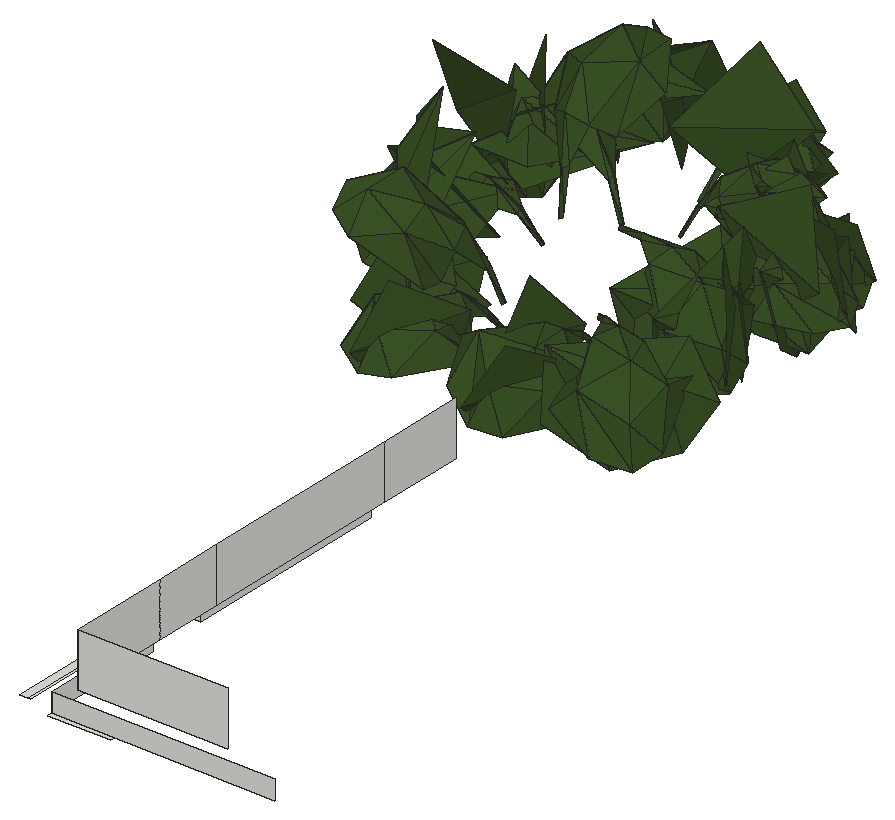
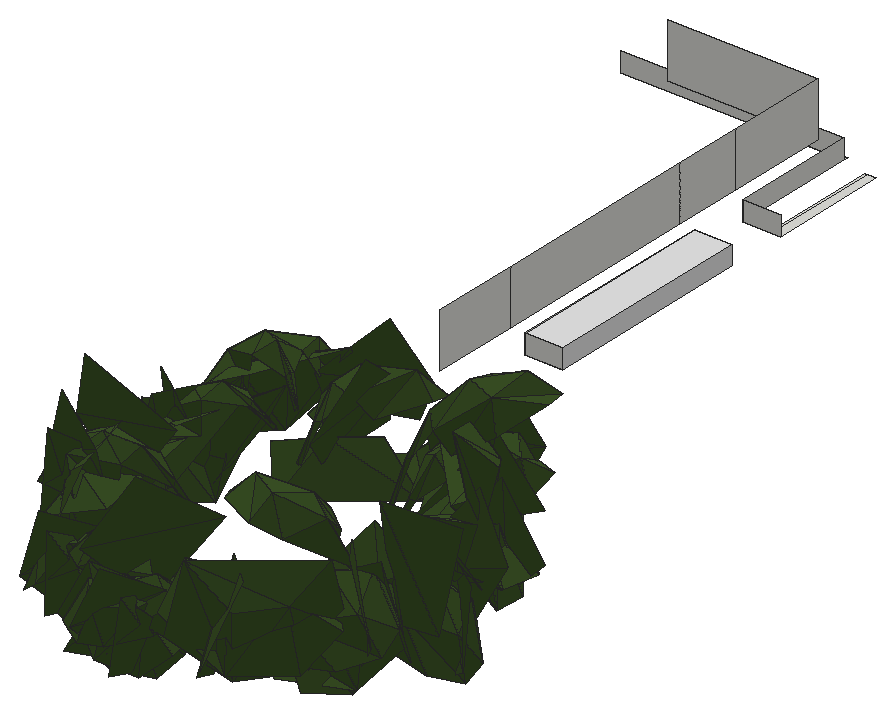
# SketchUp Ruby script. Lengths in inches.
U = 1.inch
M = Sketchup.active_model
def pt(a) = Geom::Point3d.new(a.map { |v| v * U })
def face(e, loops, mat)
  f = e.add_face(loops[0].map { |a| pt(a) })
  loops[1..].each { |l| e.add_face(l.map { |a| pt(a) }).erase! }
  f.material = f.back_material = mat if mat
  f
end
# faces: each face lists its corners as indices into pts; further lists are holes
def faces(e, pts, list, mat = nil) = list.each { |f| face(e, (f[0].is_a?(Array) ? f : [f]).map { |l| l.map { |i| pts[i] } }, mat) }
# xy, xz, yz: faces in a plane at the given z, y or x. An outline is a flat list of corners, or four numbers for a rectangle; further outlines are holes
def ring(l) = l.size == 4 ? [[l[0], l[1]], [l[2], l[1]], [l[2], l[3]], [l[0], l[3]]] : l.each_slice(2).to_a
def flat(e, list, mat, &to3) = list.each { |f| face(e, (f[0].is_a?(Array) ? f : [f]).map { |l| ring(l).map { |u, v| to3.(u, v) } }, mat) }
def xy(e, z, list, mat = nil) = flat(e, list, mat) { |x, y| [x, y, z] }
def xz(e, y, list, mat = nil) = flat(e, list, mat) { |x, z| [x, y, z] }
def yz(e, x, list, mat = nil) = flat(e, list, mat) { |y, z| [x, y, z] }
def lines(e, pts, list) = list.each { |a, b| e.add_line(pt(pts[a]), pt(pts[b])) }
# prism: a flat outline (further loops are holes) pulled along v
def prism(e, loops, v, mat = nil)
  f = face(e, loops, mat); d = Geom::Vector3d.new(v.map { |x| x * U })
  f.pushpull(f.normal.samedirection?(d) ? d.length : -d.length)
end
def box(e, o, s, mat = nil) = prism(e, [[o, [o[0] + s[0], o[1], o[2]], [o[0] + s[0], o[1] + s[1], o[2]], [o[0], o[1] + s[1], o[2]]]], [0, 0, s[2]], mat)
def at(x, y, z, deg = 0) = Geom::Transformation.translation(pt([x, y, z])) * Geom::Transformation.rotation(ORIGIN, Z_AXIS, deg.degrees)
def axes(o, x, y, z) = Geom::Transformation.new([*x, 0, *y, 0, *z, 0, *pt(o).to_a, 1])
def part(name) = M.definitions.add(name)
# library, detail: a bought-in or finely detailed component or shape, given as its bounding box
def library(name, o, s) = part(name).tap { |d| box(d.entities, o, s) }
def detail(e, o, s) = box(e.add_group.entities, o, s)
def put(e, d, t, mat = nil) = e.add_instance(d, t).tap { |i| i.material = mat if mat }
def group(e, t, mat = nil) = e.add_group.tap { |g| g.transformation = t; g.material = mat if mat }.entities
root = M.entities
M.materials.add("AM113_062_Tilia").color = [58, 81, 37]
M.materials.add("white_wall").color = [233, 233, 233]
xy(root,500.91,[[418.81,115.3125,496.21,121.6875],[371.87,130.3125,382.06,278.26],[382.06,130.3125,385.62,278.26]])
xy(root,500.91,[[371.87,353.16,418.81,615.47]],"white_wall")
xy(root,525.1,[[371.87,353.16,418.81,615.47]],"white_wall")
xz(root,121.6875,[[418.81,500.91,695.48,525.1]])
xz(root,139.5,[[436.99,525.1,622.42,592.47]])
xz(root,278.26,[[371.87,500.91,418.81,525.1]])
xz(root,353.16,[[371.87,500.91,418.81,525.1]],"white_wall")
xz(root,615.47,[[371.87,500.91,418.81,525.1]])
yz(root,371.87,[[353.16,500.91,615.47,525.1]],"white_wall")
yz(root,418.81,[[121.6875,500.91,278.26,525.1],[353.16,500.91,615.47,525.1]])
yz(root,436.99,[[139.5,525.1,266.01,592.47],[266.01,525.1,353.16,592.47],[353.16,525.1,615.47,592.47],[615.47,525.1,725.65,592.47]])
p = [[447.91,850.1875,601.09],[480.87,802.46,545.55],[524.63,854.63,485.78],[519.66,855.77,573.08],[550.76,903.55,570.88],[566.41,915.91,493.375],
  [66.82,1152.99,507.09],[97.15,1146.97,487.25],[148.3,1081.53,542.29],[70.04,1143.02,489.34],[77.07,1108.81,493.43],[83.87,1137.56,535.27],
  [126.11,1173.27,559.43],[89.64,1179.86,507.09],[141.26,1229.85,490.56],[139.06,1157.11,521.98],[139.59,1190.19,597.74],[133.73,1250.28,579.96],
  [181.97,1298.85,597.52],[140.7,1312.06,529.03],[460.33,1197.81,509.56],[504.98,1203.63,490.94],[506.78,1216.99,523.57],[521.83,1250.84,491.55],
  [530.97,1079.69,610.26],[563.39,1070.9,539.31],[530.76,1136.5,491.14],[554.3125,1134.13,573.8],[530.96,1187.11,581.77],[511.65,1204.9375,507.36],
  [507.98,1282.76,501.61],[176.48,942.12,491.66],[227.05,891.03,499.89],[227.5625,915.73,575.1875],[183.07,953.21,578.2],[189.36,1017.86,590.34],
  [136.96,999.375,548.22],[518.23,1275.49,509.68],[495.63,1265.62,492.5],[438.95,1246.59,552.56],[484.28,1275.96,572],[469.9375,1297.82,492.68],
  [415.61,1273.29,514.75],[584.43,950.18,540.22],[135.1875,1050.68,522.83],[108.03,1086.63,545.74],[350.77,1219.13,560.8],[406.07,1241.46,494.25],
  [455.94,1265.91,543.95],[342.85,1283.12,576.94],[359.62,1325.95,494.31],[374.52,1387.23,525.68],[438.95,962.3,611.65],[482.72,941.64,542.47],
  [494.35,1014.66,495.65],[498.36,1001.99,581.5],[506.32,1058.04,590.46],[507.33,1085.99,517.2],[551.23,1044.6,596.52],[525.07,1058.79,495.72],
  [471.1,1096.48,548.77],[497.1,956.03,600.03],[500.73,949.14,517.51],[474.45,1025.35,496.53],[520.47,1007.79,557.6],[516.65,1062.95,581.15],
  [481.05,1093.45,526.12],[292.87,984.37,497.8],[282.8,955.1875,535.73],[288.81,958.66,537.47],[292.6,957.64,531.31],[295.68,983.59,497.81],
  [295.23,986.83,501.03],[140.7,999.67,630.68],[79.29,1009.55,558.58],[139.35,992.91,498.89],[206.45,1053.27,524.83],[209.82,1078.24,537.58],
  [116.34,1088.94,499.17],[70.63,1078.21,589.95],[413.37,931.5,550.39],[430.11,992.57,499.42],[298.04,925.78,517.78],[472.57,943.125,530.68],
  [266.72,873.6875,541.33],[504.57,1263.71,533.37],[484.96,1291.55,519.97],[212.29,919.98,623.86],[172.99,892.09,535.71],[245.73,899.09,501.97],
  [272.37,985.95,524.2],[383.31,1336.6875,601.39],[399.96,1363.62,549.01],[345.9,1352.99,502.82],[347.39,1366.73,570.93],[288.5,1350.2,508.87],
  [301.66,1358.17,571.11],[119.21,993.93,502.99],[152.05,954.03,522.83],[143.72,999.76,578.03],[98.32,1060.89,524.86],[474.87,1070.72,588.94],
  [540.9,1059.84,553.85],[550.79,1131.46,502.96],[528.22,1123.58,584.89],[519.88,1180,585.72],[539.25,1204.4,514.64],[314.03,857.13,538.16],
  [392.29,855.66,505.11],[363.78,903.56,555.05],[454.3125,896.72,507.18],[125.51,1243.76,505.61],[113.53,1168.99,535.21],[153.61,1193.39,597.49],
  [164.9,1251.9,582.9],[236.2,1283.875,561.15],[169.13,1315.93,536.15],[154.2,1007.49,573.32],[139.42,952.86,539.93],[198.6,978.07,505.88],
  [192.15,1119.27,565.37],[140.41,1071.16,570.82],[77.11,1126.41,588.08],[145.85,1194.83,533.875],[501.82,1240.17,558.45],[507.76,824.62,581.64],
  [535.83,807.78,523.32],[570.46,833.44,508.39],[561.96,839.4375,557.13],[580.59,866.67,518.5],[256.57,1346.67,545.89],[501.45,968.14,582.11],
  [527.71,973.07,518.9],[546.71,1012.75,509.22],[541.58,1007.95,558.95],[543.09,1045.22,527.51],[453.73,1198.22,538.52],[441.48,1247.4375,579.22],
  [509.8,1257.28,577.0625],[412.52,1219.85,602.63],[451.3,1229.27,560.65],[415.82,1268.25,510.05],[416.25,1269.25,580.45],[375.79,1309.71,512.41],
  [380.42,1298.71,575.9],[560.05,1179.21,617.48],[567.94,1182.12,510.15],[494.67,1206.07,521.91],[244.54,801.95,541.64],[250.54,826.95,510.85],
  [313.74,891.83,547.15],[331.65,1233.42,542.69],[318.3125,1223.97,511.11],[316.29,1221.85,513],[332.34,1230.22,547.48],[319.3125,1221.87,511.06],
  [337.7,1228.47,547.0625],[346.8,1328.27,545.82],[162.0625,942.01,514.1],[207.12,883.25,523.55],[234.53,926.86,571.02],[202.77,974.23,570.48],
  [223.35,1041.3125,535.68],[154.67,1020.29,545.73],[552.27,999.05,521.46],[519.29,1009.6,514.2],[483.48,1061.51,605.58],[520.07,1239.02,560.28],
  [352.77,1366.97,514.57],[350.22,1344.01,577.86],[381.28,1292.62,579.47],[403.64,1343.43,559.0625],[304.94,1348.0625,573.64],[293.51,1371.11,517.46],
  [428.91,1203.51,540.99],[419.97,1193.43,539.82],[394.26,1182.37,519.06],[395.92,1183.33,515.47],[424.54,1193.28,535.56],[416.75,1196.5,537.0625],
  [394.6875,1185.0625,516.7],[514.15,1117.94,571.17],[395.73,1300.69,613.09],[361.13,1303.75,517.53],[342.05,1238.18,553.91],[421.06,1312.46,534.79],
  [260.66,1360.5,549.26],[406.07,782.48,524.875],[438.12,796.97,517.66],[415.8,801.8125,567.01],[461.07,837.3125,559.23],[485.6,869.32,522.91],
  [259.96,1266.02,621.1],[241.22,1320.45,517.69],[205.76,1390.97,556.95],[311.06,1377.46,602.9375],[316.23,1389.375,518.39],[283.73,1336.55,518.62],
  [564.89,894.8,578.39],[557.0625,942.12,564.31],[322.49,1287.52,569.46],[475.82,953,556.29],[463.74,1267.42,560.88],[424.9,1272.67,557.1],
  [400.16,778.98,545.73],[395.59,808.17,521.33],[456.04,877.73,550.25],[312.95,905.48,521.39],[307.41,909.36,558.26],[309.48,853.41,565.96],
  [346.03,875.74,534.77],[497.09,1065.1875,633.88],[558.42,1006.97,610.87],[451.05,1141.24,585.71],[145.52,1124.38,582.13],[194.92,971.05,560.45],
  [167,1082.47,523.27],[447.6,894.07,529.97],[479.07,817.625,555.37],[162.4,1086.83,559.67],[220.67,870.87,568.35],[216.7,823.06,531.56],
  [255.18,801.31,523.625],[258.8,825.63,562.98],[289.56,810.36,526.36],[252.24,868.625,554.3],[473.64,1236.38,560],[251.54,1201.92,566.37],
  [277.41,1185.12,527.79],[274.75,1187.21,523.96],[248.26,1208.15,562.98],[375.5625,838.38,597.59],[368.93,795.86,551.74],[123.55,1050.04,605.55],
  [161.14,1101.41,626.16],[100.55,1115.36,604.29],[249.58,1196.96,561.41],[273.68,1184.41,525.01],[338.44,1370.61,601.54],[382.16,1195.58,567.91],
  [437.22,1212.69,564.49],[428.72,1270.74,526.02],[400.25,1252.02,580.4375],[374.69,1289.55,575.46],[393.09,1318.31,527.3125],[497.92,1123.27,579.81],
  [359.11,1333.59,553.46],[523.44,1055.42,594.57],[495.33,1095.78,594.14],[206.23,1335.11,528.33],[153.76,1285.91,535.91],[159.85,1304.18,613.81],
  [196.51,1349.42,613.59],[255.11,1349.89,651.71],[249.16,1389.07,586.14],[242.89,922.77,528.53],[199.15,883.24,534.93],[261.47,929.36,556.48],
  [450.56,892.25,567.59],[300.94,914.56,530.04],[120.22,1213.01,638.51],[92.4,1201.34,530.6],[157.86,1151.12,533.64],[285.36,922.53,571.29],
  [214.26,1100.33,553.33],[246.18,1097.22,531.47],[248.49,1097.46,535.73],[102.42,990.41,531.83],[89.63,1062.06,551.72],[397.21,845.13,585.28],
  [394.17,856.625,542.72],[403.43,950.64,531.88],[405.93,965.66,559.1875],[213.91,1103.86,559.72],[246.98,1099.96,531.9],[211.2,1109.9375,557.1],
  [234.43,1205.14,572.13],[596.16,1132.8,559.74],[567.47,1133.92,533.77],[494.08,1177.83,586.64],[183.36,1150.55,540.33],[424.4,939.91,560.35],
  [416.32,969.85,534.7],[416.26,972.51,538.73],[426.68,1240.52,534.94],[437.26,1231.07,559.06],[128.38,1132.68,587.59],[128.24,1115.27,571.02],
  [446.99,1211.29,559.41],[413.57,970.11,535.88],[416.48,935.25,567.33],[422.15,939.46,567.76],[126.17,1256.67,582.24],[288.81,960.29,578.55],
  [294.4375,975.64,535.96],[296.8,978.73,537.64],[319.11,1274.8,562.03],[316.83,1253.25,536.34],[317.2,1250.75,539.04],[322.125,1274.15,567.01],
  [319.08,1252.64,536.36],[326.91,1276.91,565.49],[292.73,977.96,536.52],[281.54,964.77,586.78],[288.42,963.97,584.94],[139.58,1034.79,635.55],
  [443.28,1125.39,631.84],[511.12,1118.83,539.75],[583.62,1104.83,593.02],[529.04,974.14,584.79],[227.68,1150.03,584.9],[235.65,1140.25,540.24],
  [236.625,1136.35,541.29],[182.75,1131.32,568.05],[356.8,1399.57,564.1],[352.18,1378.83,540.52],[301.89,1327.64,571.92],[230.89,1147.47,590.85],
  [238.53,1140.1,540.72],[235.82,1152.15,593.35],[287.47,912.66,582.71],[90.74,1266.03,574.06],[113.82,1251.11,541.53],[179.77,1185.75,592.33],
  [323.49,891.22,578.33],[268.48,831.82,617.29],[183.19,966.11,542.08],[207.89,923.98,571.57],[174.2,959.89,622.63],[149.48,1028.09,561.62],
  [351.86,1244.66,581.375],[349.64,1265.59,572.9],[217.02,1251.48,546.0625],[179.82,1302.16,542.68],[167.84,1287.87,585.61],[114.57,1290.32,552.01],
  [538.14,1091.83,593.95],[581.26,1101.17,549.85],[592.42,1144.05,543.03],[572.27,1139.95,586.0625],[575.99,1175.04,550.97],[201.45,1354.02,543.05],
  [141.59,1309.92,546.67],[171.17,1297.21,616.98],[217.62,1330.05,622.25],[288.9,1306.23,624.27],[269.03,1372.8,598.73],[408.56,1275.59,610.93],
  [353.05,1273.15,544.59],[380.85,1295.11,590.125],[352.07,1307.71,559.67],[472.66,874.95,575.92],[436.96,802.72,616.24],[174.09,1147.3,658.14],
  [134.53,1171.67,545.81],[57.86,1201.625,571.01],[333.28,1302.43,587.63],[268.74,1327.92,594.18],[303.4375,1223.82,628.03],[347.77,1284.93,546.03],
  [396.03,1334.41,608.96],[224.79,1237.01,580.21],[118.87,1273.17,586.46],[361.8,1227.53,569.41],[319.1875,1295.16,548.27],[435.85,1035.83,626.5],
  [264.1,1305.77,560.77],[404.63,1137.39,549.54],[439.06,1133.04,581.49],[434.5,1137.9375,584.42],[402.06,1138.94,553.375],[378.35,1221.3,549.625],
  [423.72,1214.65,564.44],[416.28,1232.07,592.19],[348.33,1399.59,549.65],[345.46,1381.12,582.05],[376.11,1345.31,588.3125],[379.16,1382.6,557],
  [320.89,1392.28,552.09],[527.74,1069.46,560.36],[433.96,1142.125,578.59],[404.73,1140.3,549.75],[534.04,1182.18,598.9375],[500.76,1213.55,575.59],
  [345.89,850.79,577.12],[148.98,1061.93,594.18],[125.1,1126.9,598.61],[302.63,1316.11,551.92],[307,1313.94,581.53],[305.08,1358.79,585.4],
  [276.04,1340.03,561.28],[87.53,1251.71,559.16],[172.37,1107.69,578.08],[466.76,873.79,573.375],[443.29,995.01,589.86],[279.05,877.82,581.32],
  [184.83,1345.87,651.89],[393.43,1334.72,562.21],[533.84,875.85,602.17],[487.11,1216.65,619.08],[343.8,1298.14,581.08],[358.67,1302.8,558.56],
  [505.79,1022.07,614.51],[432.97,853.76,590.92],[386.53,903.73,632.8],[94.24,1215.87,572.36],[116.32,1252.78,598],[495.66,1186.0625,618.49],
  [569.76,1145.4375,641.81],[420.94,1307.49,568.625],[455.77,1218.04,581.08],[431.1875,899.54,591.14],[478.8125,1102.54,564.95],[202.29,1131.01,589.49],
  [216.77,1216.07,604.16],[199.78,1192.4,599.62],[140.7,1004.65,643.62],[159.27,1051.72,697.53],[114.41,1068.71,642.01],[324.64,1303.85,592.54],
  [478.41,1174.9,563.15],[479.83,1166.98,599.58],[141.34,1198.11,614.71],[158.85,1152.01,592.21],[191.94,1180.06,564.02],[294.02,1328.84,596.76],
  [337.64,1377.47,625.63],[513.41,928.66,564.21],[516.47,918.42,599.5],[450.62,1256.41,573.1875],[471.07,1117.71,595.7],[380.97,897.67,566.1],
  [404.3,903.83,587.52],[423.875,1278.77,595.51],[444.41,1291.42,569.75],[380.5,1263.18,598.5],[62.73,1157.375,670.14],[458.92,1109.3,624.52],
  [228.05,934.74,635.5],[477.26,887.39,603.98],[181.03,1181.78,627.7],[126.78,1252.57,656.33],[277.25,940.91,632.31],[282.8,915.93,618.99],
  [473.64,1141.86,611.99],[497.93,1096.4375,641.11],[171.125,1229.56,617.54],[463.39,931.38,597.95],[435.66,951.6,580.66],[433.59,951.97,585.21],
  [433.65,949.49,580.79],[461.66,920.97,599.91],[462.2,927.34,603.8],[329.47,1339.8125,598.75],[450.25,1007.56,622.8125],[178.86,1148.54,634.89],
  [152.99,1248.65,642.68],[220.4,1165.85,641.75],[197.19,1178.15,630.81],[257.24,871.625,649.35],[286.76,863.85,599.6],[273.5,906.15,585.35],
  [519.22,1146.13,614.41],[166.51,1223.77,600.87],[258.35,959.54,623.63],[461.6,1064.99,593.02],[472.22,1052.59,624.51],[546.125,1139.34,686.85],
  [246.61,1169.9375,633.07],[498.11,902.39,616.19],[207.33,846.56,638.26],[194.87,1194.61,599.58],[178.77,1222.43,668.86],[153.68,1208.9375,617.14],
  [232.29,963.21,607.04],[180.625,959.68,643.96],[200.59,939.88,672.7],[343.87,1313.49,697.67],[464.05,1028.25,637.56],[189.99,1277.78,666.25],
  [252.05,910.74,662.65],[267.75,1222.36,690.4],[265.46,1189.55,619.0625],[295.28,1228.47,661.8],[382.86,1046.72,619.66],[421.86,1031.07,628.9],
  [420.1,1036.43,634.39],[382.23,1048.31,624.66],[418.9,1041.29,629.71],[383.78,1049.47,619.99],[212.82,1201.15,678.12],[175.93,860.29,650.76],
  [203.66,880.67,674.93],[161,901.58,661.06],[262.18,1277.86,687.64],[219.48,1256.17,699.11],[220.42,1292.6,680.53]]
faces(root,p,[[0,1,2],[2,3,0],[4,3,2],[2,5,4],[6,7,8],[9,10,11],[9,11,12],[12,13,9],
  [14,15,16],[16,17,14],[14,17,18],[18,19,14],[20,21,22],[22,21,23],[24,25,26],[26,27,24],
  [28,27,26],[26,29,28],[22,23,30],[31,32,33],[33,34,31],[35,36,31],[31,34,35],[37,38,39],
  [40,41,42],[5,43,4],[10,44,45],[11,10,45],[46,47,48],[49,50,51],[52,53,54],[54,55,52],
  [56,55,54],[54,57,56],[58,59,60],[61,62,63],[63,64,61],[65,64,63],[63,66,65],[67,68,69],
  [70,71,72],[69,72,67],[73,74,75],[73,75,76],[77,78,79],[80,81,82],[80,83,81],[32,84,33],
  [72,69,70],[30,85,22],[30,86,85],[87,88,89],[87,89,90],[91,92,93],[93,94,91],[93,95,96],
  [96,94,93],[97,98,99],[100,97,99],[101,102,103],[103,104,101],[105,104,103],[103,106,105],[82,107,108],
  [108,109,82],[80,109,108],[108,110,80],[111,112,113],[113,114,111],[115,116,111],[111,114,115],[117,118,119],
  [117,119,120],[8,121,6],[121,122,6],[12,123,13],[110,83,80],[29,124,28],[125,126,127],[127,128,125],
  [127,129,128],[95,130,96],[131,132,133],[133,134,131],[133,135,134],[22,136,20],[39,137,37],[137,138,37],
  [139,140,141],[141,142,139],[141,143,144],[144,142,141],[145,146,147],[148,149,150],[151,152,153],[154,153,155],
  [155,156,154],[143,157,144],[153,154,151],[158,159,160],[160,161,158],[162,163,158],[158,161,162],[164,165,166],
  [106,167,105],[168,169,170],[170,171,168],[172,169,168],[168,173,172],[40,42,174],[175,176,177],[177,178,175],
  [179,180,176],[57,181,56],[182,183,184],[182,185,183],[173,186,172],[187,188,189],[189,188,190],[188,191,190],
  [192,193,194],[82,109,80],[195,196,197],[128,129,198],[129,199,198],[195,197,200],[131,201,132],[176,175,179],
  [85,86,202],[86,203,202],[204,205,206],[207,208,209],[209,210,207],[166,211,164],[211,212,164],[145,147,213],
  [15,214,16],[99,98,215],[45,44,216],[190,191,217],[125,218,126],[216,219,45],[220,221,222],[222,223,220],
  [222,224,223],[159,225,160],[136,22,226],[22,85,226],[227,228,229],[229,230,227],[231,232,187],[187,189,231],
  [99,233,100],[100,233,234],[234,235,100],[236,237,228],[238,49,51],[239,240,241],[241,242,239],[243,242,241],
  [241,244,243],[66,245,65],[223,224,209],[224,210,209],[244,246,243],[134,135,247],[135,248,247],[228,227,236],
  [249,250,251],[251,252,249],[249,252,253],[253,254,249],[255,256,220],[220,257,255],[217,258,190],[160,225,259],
  [160,259,162],[260,261,262],[263,208,70],[70,69,263],[264,265,266],[220,256,221],[267,118,117],[268,267,117],
  [269,270,271],[271,272,269],[273,266,274],[274,275,273],[226,85,202],[260,262,276],[277,278,279],[280,123,12],
  [281,282,283],[284,285,202],[202,203,284],[112,286,113],[287,11,45],[12,11,287],[288,175,178],[178,136,288],
  [68,257,263],[263,69,68],[162,161,160],[266,273,264],[289,290,291],[291,283,289],[250,292,251],[293,294,295],
  [296,297,298],[299,298,300],[300,301,299],[302,303,304],[304,295,302],[179,175,288],[288,285,179],[295,304,293],
  [305,77,79],[226,288,136],[283,291,281],[298,299,296],[306,307,308],[4,43,309],[310,311,312],[12,313,280],
  [314,315,316],[317,312,318],[318,319,317],[33,84,320],[312,317,310],[321,322,323],[150,324,148],[324,325,148],
  [326,327,328],[329,326,328],[151,154,330],[330,331,151],[332,333,334],[334,333,335],[336,337,338],[338,339,336],
  [338,340,339],[341,342,343],[343,344,341],[345,346,341],[341,344,345],[347,46,48],[348,331,349],[349,350,348],
  [206,351,204],[351,352,204],[287,45,219],[353,354,355],[144,157,356],[96,130,357],[358,359,360],[334,361,332],
  [342,362,343],[156,363,330],[330,154,156],[243,364,239],[243,246,364],[58,60,365],[172,186,366],[367,368,369],
  [369,370,367],[371,372,373],[373,363,371],[374,375,376],[376,377,374],[374,378,375],[336,379,337],[380,381,370],
  [339,340,382],[340,383,382],[231,384,232],[117,385,268],[268,385,120],[120,386,268],[387,388,389],[389,390,387],
  [334,335,391],[378,390,389],[375,378,389],[392,219,264],[264,273,392],[370,369,380],[393,218,125],[394,201,131],
  [257,220,395],[395,263,257],[396,192,194],[376,397,377],[125,128,398],[398,128,198],[392,273,275],[275,313,392],
  [61,64,65],[395,209,208],[395,208,263],[28,124,399],[376,400,401],[401,397,376],[131,134,402],[402,134,247],
  [226,285,288],[226,202,285],[403,189,190],[403,190,258],[272,404,269],[391,405,406],[391,406,334],[313,12,287],
  [287,219,392],[279,407,277],[407,408,277],[409,350,349],[105,167,410],[411,258,281],[281,291,411],[99,215,234],
  [412,379,336],[172,366,170],[113,413,115],[115,114,113],[414,415,236],[236,227,414],[328,416,329],[329,416,417],
  [417,418,329],[296,299,419],[419,388,296],[220,223,395],[395,223,209],[414,227,230],[230,361,414],[420,421,382],
  [382,383,420],[422,423,424],[424,415,422],[316,425,314],[425,426,314],[198,199,427],[427,428,198],[373,372,429],
  [336,430,412],[120,385,117],[419,299,301],[301,400,419],[431,384,231],[231,432,431],[231,189,403],[290,432,411],
  [411,291,290],[403,258,411],[239,242,243],[287,392,313],[433,409,349],[434,409,433],[435,330,363],[363,373,435],
  [373,429,434],[434,433,373],[4,309,0],[0,3,4],[91,94,96],[436,353,355],[96,357,91],[56,181,437],
  [328,327,438],[405,423,422],[406,405,422],[435,331,330],[435,349,331],[125,439,393],[170,169,172],[24,27,28],
  [323,440,321],[440,441,321],[33,320,35],[35,34,33],[144,356,139],[139,142,144],[234,233,99],[398,198,428],
  [442,443,293],[293,304,442],[380,369,444],[444,421,380],[65,245,445],[18,17,16],[446,414,361],[361,334,446],
  [447,448,449],[450,451,452],[452,449,450],[105,410,101],[453,419,400],[400,376,453],[65,445,61],[52,55,56],
  [368,430,444],[444,369,368],[453,388,419],[453,389,388],[439,125,398],[28,399,24],[131,454,394],[454,131,402],
  [16,214,455],[453,375,389],[376,375,453],[251,292,456],[442,304,303],[101,104,105],[310,317,457],[457,458,310],
  [449,452,447],[459,460,461],[461,443,459],[334,406,446],[336,339,462],[462,339,382],[343,362,463],[303,464,442],
  [432,231,403],[403,411,432],[113,286,413],[435,433,349],[56,437,52],[457,317,319],[373,433,435],[465,466,247],
  [247,248,465],[467,306,308],[319,468,457],[430,336,462],[402,247,466],[462,444,430],[16,455,18],[447,452,469],
  [469,428,447],[446,406,422],[462,382,421],[398,428,469],[470,460,459],[462,421,444],[471,458,472],[446,422,415],
  [446,415,414],[472,473,471],[451,439,469],[469,452,451],[343,463,345],[398,469,439],[474,475,476],[476,464,474],
  [477,358,360],[253,252,251],[251,456,253],[402,478,454],[402,466,478],[345,344,343],[479,473,472],[480,459,443],
  [480,443,442],[481,468,482],[482,483,481],[484,485,486],[486,487,484],[488,489,487],[328,438,417],[417,416,328],
  [485,454,478],[464,476,480],[480,442,464],[478,466,488],[487,486,488],[478,486,485],[488,486,478],[490,458,457],
  [490,472,458],[490,457,468],[468,481,490],[491,470,492],[492,470,459],[476,475,493],[480,492,459],[476,493,491],
  [491,492,476],[481,483,494],[476,492,480],[495,479,472],[496,479,495],[490,495,472],[481,495,490],[496,495,481],
  [481,494,496]],"AM113_062_Tilia")
